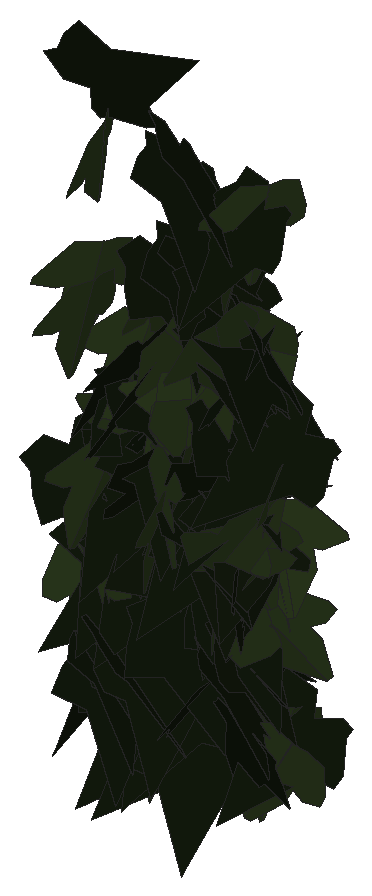
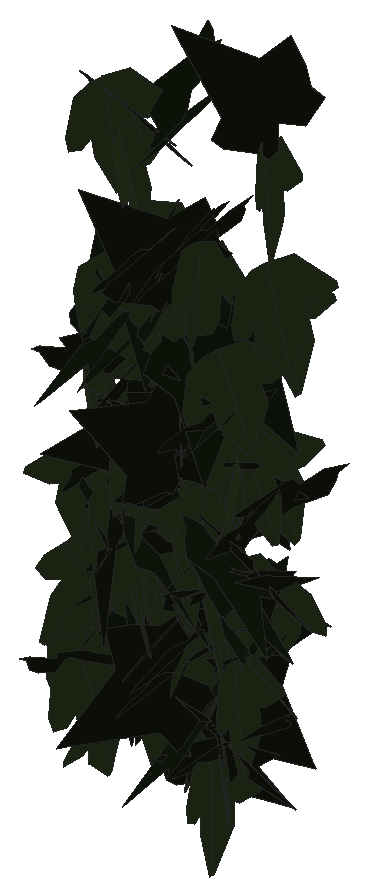
# SketchUp Ruby script. Lengths in inches.
U = 1.inch
M = Sketchup.active_model
def pt(a) = Geom::Point3d.new(a.map { |v| v * U })
def face(e, loops, mat)
  f = e.add_face(loops[0].map { |a| pt(a) })
  loops[1..].each { |l| e.add_face(l.map { |a| pt(a) }).erase! }
  f.material = f.back_material = mat if mat
  f
end
# faces: each face lists its corners as indices into pts; further lists are holes
def faces(e, pts, list, mat = nil) = list.each { |f| face(e, (f[0].is_a?(Array) ? f : [f]).map { |l| l.map { |i| pts[i] } }, mat) }
# xy, xz, yz: faces in a plane at the given z, y or x. An outline is a flat list of corners, or four numbers for a rectangle; further outlines are holes
def ring(l) = l.size == 4 ? [[l[0], l[1]], [l[2], l[1]], [l[2], l[3]], [l[0], l[3]]] : l.each_slice(2).to_a
def flat(e, list, mat, &to3) = list.each { |f| face(e, (f[0].is_a?(Array) ? f : [f]).map { |l| ring(l).map { |u, v| to3.(u, v) } }, mat) }
def xy(e, z, list, mat = nil) = flat(e, list, mat) { |x, y| [x, y, z] }
def xz(e, y, list, mat = nil) = flat(e, list, mat) { |x, z| [x, y, z] }
def yz(e, x, list, mat = nil) = flat(e, list, mat) { |y, z| [x, y, z] }
def lines(e, pts, list) = list.each { |a, b| e.add_line(pt(pts[a]), pt(pts[b])) }
# prism: a flat outline (further loops are holes) pulled along v
def prism(e, loops, v, mat = nil)
  f = face(e, loops, mat); d = Geom::Vector3d.new(v.map { |x| x * U })
  f.pushpull(f.normal.samedirection?(d) ? d.length : -d.length)
end
def box(e, o, s, mat = nil) = prism(e, [[o, [o[0] + s[0], o[1], o[2]], [o[0] + s[0], o[1] + s[1], o[2]], [o[0], o[1] + s[1], o[2]]]], [0, 0, s[2]], mat)
def at(x, y, z, deg = 0) = Geom::Transformation.translation(pt([x, y, z])) * Geom::Transformation.rotation(ORIGIN, Z_AXIS, deg.degrees)
def axes(o, x, y, z) = Geom::Transformation.new([*x, 0, *y, 0, *z, 0, *pt(o).to_a, 1])
def part(name) = M.definitions.add(name)
# library, detail: a bought-in or finely detailed component or shape, given as its bounding box
def library(name, o, s) = part(name).tap { |d| box(d.entities, o, s) }
def detail(e, o, s) = box(e.add_group.entities, o, s)
def put(e, d, t, mat = nil) = e.add_instance(d, t).tap { |i| i.material = mat if mat }
def group(e, t, mat = nil) = e.add_group.tap { |g| g.transformation = t; g.material = mat if mat }.entities
root = M.entities
M.materials.add("efeu1").color = [18, 25, 13]
M.materials.add("efeu2").color = [43, 57, 29]
c1 = part("ivyleaf_10")
p = [[0,0.5,-0.03],[-0.0625,2.02,-0.43],[-0.19,2.01,-0.46],[-0.54,1.05,-0.29],[-0.52,0.625,-0.18],[-0.83,0.76,-0.28],
  [-1.16,0.64,-0.33],[-1.15,0.33,-0.24],[-0.77,-0.39,0.02],[-0.3,-0.51,0.16],[0.04,-0.48,0.23],[-0.02,2.01,-0.4375],
  [-0.06,2.01,-0.43],[0.04,-0.49,0.23],[0.67,-0.49,0.14],[1.38,0.36,-0.2],[1.375,0.51,-0.24],[0.81,0.65,-0.19],
  [0.62,0.59,-0.15],[0.6,1.09,-0.28],[0.5,1.23,-0.31]]
faces(c1.entities,p,[[0,1,2,3,4,5,6,7,8,9,10],[11,12,0,13,14,15,16,17,18,19,20]],"efeu2")
c2 = part("ivyleaf_9")
p = [[1.54,2.16,1.25],[1.36,2.04,1.19],[-0.21,0.99,0.68],[-0.71,1.11,0.82],[-0.85,0.86,0.67],[-0.8,0.17,0.21],
  [-0.9,-0.01,0.1],[-0.67,-0.16,-0.02],[-0.08,-0.08,-0.05],[-0.03,-0.6,-0.4],[0.65,-0.88,-0.66],[0.83,-0.6,-0.49],
  [1.29,-0.42,-0.43],[1.8125,-0.07,-0.26],[1.21,0.44,0.15]]
faces(c2.entities,p,[[0,1,2,3,4,5,6,7,8,9,10,11,12,13,14]],"efeu1")
put(root,c1,axes([34.11,223.34,234.7],[0.03358,-0.4914,-0.086],[-0.00003,0.0862,-0.49251],[0.49887,0.03309,0.00576]))
put(root,c1,axes([34.14,222.76,239.2],[-0.18902,-0.45532,0.08338],[0.00238,-0.09102,-0.49164],[0.46289,-0.18546,0.03657]))
put(root,c2,axes([34.125,223.26,234.54],[-0.15536,0.18817,-0.43641],[0.22397,-0.37597,-0.24184],[-0.41916,-0.27063,0.03253]))
put(root,c2,axes([33.87,222.69,236.875],[0.17375,-0.38611,-0.26595],[0.02805,0.29168,-0.40514],[0.468,0.12586,0.12302]))
put(root,c1,axes([34.16,222.77,240.65],[0.12089,-0.4627,-0.14593],[-0.00592,0.14897,-0.47726],[0.48513,0.11712,0.03054]))
put(root,c2,axes([34.42,223.24,236.16],[-0.17172,0.43146,0.18535],[-0.15176,0.13578,-0.45666],[-0.44439,-0.21309,0.08432]))
put(root,c1,axes([34.19,222.53,238.87],[-0.0271,-0.49787,0.03732],[0.00573,-0.03768,-0.49855],[0.49923,-0.02659,0.00774]))
put(root,c1,axes([34.2,223.65,233.7],[0.00023,-0.48904,-0.10413],[0.02345,0.10403,-0.4885],[0.49945,-0.00466,0.02298]))
put(root,c2,axes([34.56,223.33,233.95],[-0.28419,0.24786,0.32834],[-0.27435,0.18318,-0.37574],[-0.30655,-0.39372,0.03188]))
put(root,c1,axes([34.41,222.93,237.19],[-0.43307,-0.01374,0.24952],[-0.24213,-0.1004,-0.42578],[0.0618,-0.48962,0.08031]))
put(root,c1,axes([34.23,223.51,234.2],[0.28638,-0.40282,-0.07567],[0.00576,0.09625,-0.49061],[0.40982,0.28013,0.05977]))
put(root,c1,axes([34.08,222.67,235.6],[0.47852,-0.03633,0.14036],[0.13956,-0.01571,-0.47987],[0.03928,0.49843,-0.0049]))
put(root,c2,axes([34.03,223.48,234.11],[0.07427,-0.47912,-0.12219],[0.08679,0.13427,-0.47375],[0.48678,0.04916,0.10311]))
put(root,c2,axes([34.5,223.35,236.12],[-0.39406,0.27061,-0.14658],[0.08038,-0.13938,-0.4734],[-0.29708,-0.39667,0.06634]))
put(root,c1,axes([34.36,222.62,236.94],[-0.08972,-0.4571,0.18168],[-0.00274,-0.18421,-0.46482],[0.49188,-0.0844,0.03055]))
put(root,c2,axes([34.11,223.26,236.59],[0.07666,-0.49409,0.00124],[0.00011,-0.00124,-0.5],[0.49409,0.07666,-0.00008]))
put(root,c2,axes([34.29,223.24,235.73],[-0.30239,-0.39405,0.05729],[0.056,-0.11331,-0.48376],[0.39424,-0.28615,0.11266]))
put(root,c1,axes([34.44,223.18,238.26],[-0.26244,-0.39372,0.16159],[-0.00493,-0.18701,-0.46368],[0.42556,-0.24497,0.09428]))
put(root,c2,axes([34.5625,223.14,235.54],[-0.38086,-0.25859,0.19513],[-0.15815,-0.11442,-0.46032],[0.28272,-0.41236,0.00536]))
put(root,c2,axes([34.56,223.5,233.75],[-0.4195,-0.25933,0.08226],[-0.05676,-0.06442,-0.49257],[0.26608,-0.42261,0.02461]))
put(root,c1,axes([34.51,223.36,235.55],[0.30708,-0.35032,-0.18159],[-0.09709,0.15595,-0.46503],[0.38246,0.32087,0.02776]))
put(root,c2,axes([34.75,223.04,236.17],[-0.48681,0.10802,0.03673],[-0.03736,0.00117,-0.4986],[-0.1078,-0.48819,0.00693]))
put(root,c1,axes([34.51,223.0625,236.9],[-0.38778,0.31246,0.04468],[-0.03268,0.03066,-0.49799],[-0.31394,-0.38914,-0.00335]))
put(root,c2,axes([34.11,222.76,241.23],[0.03647,-0.07809,0.49252],[0.46778,-0.16576,-0.06092],[0.17279,0.46522,0.06097]))
put(root,c2,axes([34.72,222.96,235.22],[-0.4416,0.2098,-0.10473],[0.08598,-0.06289,-0.48852],[-0.21816,-0.44947,0.01946]))
put(root,c2,axes([34.3125,222.74,234.62],[0.14282,-0.45162,0.16012],[0.06793,-0.14631,-0.47326],[0.47433,0.15694,0.01957]))
put(root,c2,axes([34.76,222.69,238.39],[-0.19998,0.38391,-0.25024],[0.05685,-0.25014,-0.42918],[-0.45473,-0.20011,0.05639]))
put(root,c2,axes([34.63,223.28,235.65],[-0.31388,-0.37861,0.0902],[0.01511,-0.12764,-0.4832],[0.38891,-0.3006,0.09157]))
put(root,c2,axes([34.69,222.86,236.79],[-0.4249,-0.2517,-0.07816],[0.07005,0.0351,-0.49382],[0.25408,-0.4306,0.00543]))
put(root,c2,axes([34.42,223.43,236.28],[0.04909,-0.47702,0.14157],[0.07836,-0.13307,-0.47556],[0.49138,0.06887,0.06169]))
put(root,c1,axes([34.67,223,234.7],[-0.20063,-0.44955,-0.08745],[0.07749,0.06078,-0.4902],[0.45138,-0.21025,0.04529]))
put(root,c2,axes([34.47,223.54,234.28],[0.37542,-0.29256,-0.1532],[-0.08783,0.13514,-0.47331],[0.31835,0.38229,0.05007]))
put(root,c2,axes([34.5625,222.63,234.59],[-0.04459,-0.49779,-0.01458],[0.00178,0.01448,-0.49979],[0.498,-0.04462,0.00048]))
put(root,c2,axes([34.48,223.23,234.26],[0.06732,-0.45206,0.20277],[0.083,-0.19145,-0.45438],[0.48845,0.09483,0.04926]))
put(root,c1,axes([34.6,223.14,236.6],[0.21448,0.43607,0.11765],[0.04232,0.11026,-0.48585],[-0.44967,0.21837,0.01039]))
put(root,c2,axes([34.6,223.01,237.6],[0.03646,-0.46071,-0.19083],[0.04023,0.19343,-0.45931],[0.49704,0.01813,0.05118]))
put(root,c1,axes([34.81,223.26,236.66],[0.4838,-0.10925,-0.06327],[-0.05445,0.0455,-0.49494],[0.1139,0.48579,0.03213]))
put(root,c2,axes([34.53,222.91,237.75],[0.28843,-0.40826,0.01141],[0.08787,0.04839,-0.48983],[0.39886,0.28457,0.09966]))
put(root,c2,axes([34.55,222.39,235.01],[0.39792,-0.29941,0.04482],[0.03562,-0.02722,-0.49799],[0.30065,0.39951,-0.00033]))
put(root,c1,axes([34.61,222.62,237.51],[-0.12944,-0.16385,-0.45431],[0.37363,0.26406,-0.20169],[0.30602,-0.3917,0.05408]))
put(root,c1,axes([35.01,222.91,235.2],[-0.47143,-0.05851,0.15599],[-0.13811,-0.12462,-0.46411],[0.09319,-0.48067,0.10134]))
put(root,c2,axes([34.96,221.96,237.88],[0.08046,0.31546,0.37949],[0.03899,0.37923,-0.32352],[-0.49194,0.08166,0.03643]))
put(root,c1,axes([34.98,222.88,239.2],[-0.0234,-0.47311,-0.16006],[0.00964,0.15978,-0.47369],[0.49936,-0.02526,0.00165]))
put(root,c2,axes([34.73,222.58,236.74],[0.24245,0.18452,0.39645],[0.29624,0.26412,-0.3041],[-0.32165,0.38235,0.01875]))
put(root,c2,axes([35.07,223.15,233.89],[-0.38153,-0.2921,0.13824],[-0.07227,-0.13135,-0.477],[0.31498,-0.38396,0.05801]))
put(root,c2,axes([35.09,223.14,237.37],[-0.06976,0.2846,-0.40513],[0.04835,-0.40327,-0.29162],[-0.49274,-0.07986,0.02874]))
put(root,c2,axes([35.17,222.66,237.82],[-0.03634,0.4743,0.154],[-0.07238,0.14776,-0.47215],[-0.4934,-0.05661,0.05792]))
put(root,c2,axes([34.77,223.41,235.01],[0.13319,-0.47341,-0.09026],[-0.00605,0.09199,-0.49143],[0.4819,0.132,0.01878]))
put(root,c2,axes([35.09,223.06,234.37],[-0.40654,-0.28505,-0.05895],[0.04738,0.03512,-0.49651],[0.2872,-0.40929,-0.00154]))
put(root,c1,axes([35.1,223.18,236.1],[0.46743,-0.01759,-0.17663],[-0.15297,0.21249,-0.42597],[0.09005,0.45226,0.19326]))
put(root,c1,axes([35.08,222.72,233.96],[0.13868,-0.35633,-0.32217],[-0.01819,0.33119,-0.37414],[0.48004,0.1155,0.07889]))
put(root,c1,axes([34.86,223.04,235.77],[0.28357,-0.32752,0.24963],[0.24765,-0.10654,-0.42109],[0.32903,0.36246,0.1018]))
put(root,c2,axes([34.8125,223.5,234.63],[0.42765,0.17333,0.19253],[0.1735,0.08432,-0.46129],[-0.19238,0.46135,0.01198]))
put(root,c2,axes([34.89,223.44,234.61],[0.09393,-0.4685,-0.14725],[-0.00409,0.14916,-0.47721],[0.49108,0.09085,0.02418]))
put(root,c1,axes([35.2,223.22,234.41],[-0.40893,-0.28756,-0.00917],[0.0055,0.00813,-0.4999],[0.28766,-0.40895,-0.00348]))
put(root,c1,axes([35.16,222.61,236.73],[0.19148,-0.4548,0.08061],[0.04294,-0.06935,-0.4933],[0.45988,0.19583,0.0125]))
put(root,c2,axes([35.01,223.38,237.2],[0.07138,-0.05001,0.49235],[0.35069,0.35609,-0.01467],[-0.34918,0.34741,0.08591]))
put(root,c1,axes([35.04,222.58,237.1],[-0.34113,0.24052,-0.27529],[0.16592,-0.23364,-0.40973],[-0.32573,-0.37089,0.07959]))
put(root,c1,axes([35.2,222.94,237.29],[0.22936,-0.41378,-0.16179],[-0.00212,0.18105,-0.46606],[0.44428,0.21448,0.0813]))
put(root,c2,axes([35.13,222.71,234.87],[-0.31475,-0.33373,-0.1989],[0.13584,0.14528,-0.45874],[0.36398,-0.34281,-0.00079]))
put(root,c2,axes([35.12,222.89,237.35],[-0.27304,-0.38906,-0.15519],[0.12237,0.10307,-0.47371],[0.40059,-0.29666,0.03894]))
put(root,c2,axes([35.49,223.23,236.07],[-0.34253,0.36424,0.0015],[-0.00669,-0.00424,-0.49994],[-0.36418,-0.34251,0.00778]))
put(root,c1,axes([35.33,223.25,235.84],[-0.33116,-0.36474,0.08542],[-0.0186,-0.09786,-0.48998],[0.37415,-0.3277,0.05125]))
put(root,c2,axes([35.12,222.92,236.1],[-0.14947,-0.43464,-0.19685],[0.06943,0.18428,-0.45959],[0.47206,-0.16472,0.00527]))
put(root,c2,axes([35.03,222.75,239.53],[0.18427,-0.43161,-0.1725],[-0.01394,0.18034,-0.46613],[0.4646,0.1766,0.05443]))
put(root,c1,axes([35.53,222.6875,238.05],[-0.3951,0.00452,0.3064],[-0.29003,-0.16686,-0.37154],[0.0989,-0.47131,0.13447]))
put(root,c2,axes([35.48,223.25,235.79],[-0.47885,-0.13396,0.0525],[-0.05066,-0.0138,-0.49724],[0.13467,-0.48152,-0.00035]))
put(root,c2,axes([35.06,223.27,235.0625],[0.19502,-0.45951,-0.02855],[0.00677,0.03386,-0.49881],[0.46035,0.19417,0.01943]))
put(root,c1,axes([35.39,223.29,236.17],[0.13846,-0.46313,-0.12785],[-0.00092,0.13279,-0.48204],[0.48045,0.13372,0.03592]))
put(root,c2,axes([35.17,223.07,239.39],[0.07597,-0.48494,0.09521],[-0.0029,-0.09677,-0.49054],[0.49419,0.07398,-0.01751]))
put(root,c2,axes([35.3,223.02,233.86],[-0.23079,-0.429,-0.11267],[0.08281,0.0831,-0.48604],[0.43575,-0.243,0.03269]))
put(root,c2,axes([35.21,223.16,234.57],[0.49727,-0.03058,-0.04225],[-0.04176,0.00925,-0.49817],[0.03125,0.49898,0.00664]))
put(root,c1,axes([35.38,222.49,238.8125],[-0.14094,-0.3639,-0.31259],[0.16426,0.2695,-0.3878],[0.45073,-0.21201,0.04358]))
put(root,c1,axes([35.54,222.81,235.83],[0.3514,-0.27279,-0.22825],[-0.10366,0.22839,-0.43254],[0.34025,0.35132,0.10396]))
put(root,c2,axes([35.54,223.03,236.4375],[-0.43177,-0.25164,-0.01603],[0.06393,-0.0785,-0.48964],[0.24391,-0.42487,0.09996]))
put(root,c1,axes([35.44,223.37,235.26],[0.3071,-0.39402,0.02088],[0.0456,0.00916,-0.49783],[0.39193,0.30767,0.04156]))
put(root,c1,axes([35.37,222.5,238.11],[-0.03035,-0.1272,-0.48259],[0.27004,0.40241,-0.12305],[0.41971,-0.26811,0.04427]))
put(root,c2,axes([35.71,223.09,237.34],[-0.47637,-0.15158,0.00989],[-0.00928,-0.00346,-0.4999],[0.15162,-0.47646,0.00049]))
put(root,c2,axes([35.33,222.92,239.02],[-0.10944,-0.07824,0.48156],[0.47076,0.11265,0.12529],[-0.1281,0.48082,0.04901]))
put(root,c2,axes([35.45,223.3,236],[-0.09988,-0.48477,0.07083],[0.00562,-0.07342,-0.49455],[0.48989,-0.09799,0.02012]))
put(root,c2,axes([35.17,223.23,234.93],[0.27037,-0.243,0.34329],[0.26826,-0.21469,-0.36324],[0.32395,0.3806,0.01428]))
put(root,c2,axes([35.4,222.58,235.47],[0.03156,-0.45448,-0.20603],[0.03565,0.20797,-0.4533],[0.49773,0.01392,0.04554]))
put(root,c2,axes([35.36,223.24,235.09],[0.26801,-0.3956,-0.14722],[-0.01015,0.16829,-0.47072],[0.42198,0.25531,0.08218]))
put(root,c2,axes([35.38,222.68,240.68],[0.05009,-0.46932,0.16501],[0.08782,-0.1549,-0.46722],[0.48967,0.07579,0.06691]))
put(root,c2,axes([35.8125,222.49,234.89],[-0.19665,0.45294,-0.07859],[0.02413,-0.07519,-0.49372],[-0.45907,-0.19797,0.00772]))
put(root,c1,axes([35.68,223.2,236.73],[0.05466,-0.49654,-0.02149],[-0.01417,0.02005,-0.4994],[0.4968,0.0552,-0.01188]))
put(root,c2,axes([35.3,222.89,236.48],[0.21085,-0.42989,0.144],[0.1583,-0.07901,-0.46765],[0.42483,0.2428,0.10278]))
put(root,c1,axes([36.05,223.23,238.57],[-0.08394,-0.00248,-0.4929],[-0.477,-0.12558,0.08186],[-0.1242,0.48397,0.01871]))
put(root,c2,axes([35.89,223.36,236.14],[0.1905,0.03593,-0.46089],[-0.45956,0.06874,-0.1846],[0.0501,0.49395,0.05921]))
put(root,c1,axes([35.76,223.25,236.39],[-0.12369,-0.4558,0.16417],[0.01058,-0.17193,-0.46939],[0.48434,-0.11265,0.05218]))
put(root,c2,axes([35.42,222.55,241.02],[0.25946,-0.38335,0.18901],[0.1003,-0.16032,-0.46286],[0.41547,0.2781,-0.00629]))
put(root,c2,axes([35.63,223.01,236.54],[-0.12405,-0.46902,-0.12095],[0.04812,0.11231,-0.48484],[0.48197,-0.13193,0.01727]))
put(root,c1,axes([35.875,222.76,236.67],[-0.4902,0.04785,0.0861],[-0.09629,-0.14065,-0.47005],[-0.02076,-0.47742,0.1471]))
put(root,c1,axes([35.71,223.5625,233.9375],[-0.01299,0.48038,-0.13807],[-0.00656,-0.13827,-0.48046],[-0.49979,-0.01067,0.00989]))
put(root,c2,axes([35.54,223.06,239.28],[0.15007,-0.4533,-0.14833],[0.01567,0.1601,-0.47342],[0.47669,0.13744,0.06226]))
put(root,c2,axes([35.46,222.67,236.94],[0.29975,0.11694,0.38272],[0.34263,0.17207,-0.32093],[-0.20677,0.45466,0.02302]))
put(root,c1,axes([35.72,223.05,235.97],[0.36094,-0.32374,0.12214],[0.08174,-0.09173,-0.48467],[0.33622,0.36984,-0.01329]))
put(root,c2,axes([36.0625,222.56,238.41],[-0.07122,0.41135,0.27517],[-0.09393,0.26172,-0.41555],[-0.48591,-0.11088,0.04]))
put(root,c2,axes([35.98,222.85,236.18],[0.11385,-0.05936,-0.48323],[-0.42227,0.23497,-0.12835],[0.24233,0.43734,0.00337]))
put(root,c2,axes([35.68,222.69,238.64],[0.42435,-0.16301,-0.20821],[-0.15674,0.16203,-0.4463],[0.21297,0.44404,0.08641]))
put(root,c2,axes([35.91,223.05,237.21],[-0.45598,-0.11059,-0.17277],[0.19559,-0.10745,-0.44744],[0.06184,-0.47563,0.14125]))
put(root,c2,axes([35.64,223.1875,235.49],[0.09036,-0.48578,-0.07651],[0.08791,0.09249,-0.48344],[0.48385,0.07392,0.10212]))
put(root,c1,axes([35.96,223.16,235.82],[-0.03905,-0.45391,-0.20601],[0.02519,0.20458,-0.45554],[0.49784,-0.04595,0.00689]))
put(root,c1,axes([36.01,222.39,239.11],[-0.12783,-0.45508,-0.16298],[0.03207,0.16022,-0.47255],[0.48232,-0.13126,-0.01178]))
put(root,c2,axes([35.76,222.89,237.81],[0.21009,-0.43728,-0.12104],[-0.0273,0.12096,-0.48438],[0.4529,0.21014,0.02695]))
put(root,c1,axes([36.03,222.8,240.16],[0.15394,-0.47571,-0.00042],[0.00298,0.0014,-0.49999],[0.4757,0.15393,0.00327]))
put(root,c2,axes([36.21,223.04,236.11],[-0.38319,0.30335,-0.10557],[0.08986,-0.05654,-0.4886],[-0.30837,-0.39342,-0.01119]))
put(root,c2,axes([35.79,223.08,235.18],[0.27184,-0.40706,-0.10202],[-0.04567,0.09213,-0.48931],[0.41715,0.27535,0.01291]))
put(root,c2,axes([35.98,223.16,236.67],[-0.18664,-0.46177,0.04398],[-0.00048,-0.04722,-0.49777],[0.46386,-0.18585,0.01718]))
put(root,c2,axes([35.83,223.2,238.47],[0.39276,-0.2591,-0.16914],[-0.09366,0.16094,-0.46403],[0.2949,0.39619,0.07789]))
put(root,c1,axes([36.14,223.36,234.12],[-0.17326,-0.45238,0.12382],[-0.01504,-0.12657,-0.48348],[0.46878,-0.17126,0.03025]))
put(root,c1,axes([36.0625,222.77,235.48],[0.05471,-0.20049,0.45476],[-0.07686,0.44859,0.20702],[-0.49102,-0.09256,0.01827]))
put(root,c1,axes([36.09,222.67,236.62],[-0.36468,-0.3089,-0.14695],[0.1142,0.09253,-0.47791],[0.32244,-0.38213,0.00307]))
put(root,c1,axes([36.05,223.24,235.41],[-0.35274,-0.23329,-0.26674],[0.21681,0.15561,-0.42282],[0.2803,-0.41395,-0.00862]))
put(root,c2,axes([36.3,222.43,234.49],[0.29551,0.10361,-0.38979],[-0.38708,-0.06291,-0.31018],[-0.11332,0.48509,0.04303]))
put(root,c1,axes([36.05,222.56,236.4],[-0.26492,-0.37221,0.20317],[0.17316,0.12372,0.45245],[-0.38709,0.31008,0.06335]))
put(root,c2,axes([36.03,223.24,238.54],[-0.06121,-0.20039,0.45398],[0.16839,-0.43867,-0.17092],[0.46679,0.13197,0.12119]))
put(root,c1,axes([36.17,223.19,236.5625],[0.36389,0.32989,0.09355],[0.03551,0.09943,-0.48873],[-0.34106,0.36233,0.04893]))
put(root,c1,axes([36.35,222.75,240.65],[-0.18862,-0.45949,0.05734],[0.01202,-0.06676,-0.49538],[0.4629,-0.1855,0.03623]))
put(root,c2,axes([36.05,222.76,238.76],[0.04886,-0.41764,0.27053],[0.13652,-0.25015,-0.41084],[0.47851,0.11401,0.08959]))
put(root,c2,axes([35.99,222.64,234.89],[0.1633,-0.37153,0.29205],[0.16539,-0.24453,-0.40355],[0.4427,0.2284,0.04303]))
put(root,c1,axes([36.32,223.03,237.3],[0.23641,-0.44042,-0.01177],[0.01527,0.02154,-0.4993],[0.44031,0.23572,0.02364]))
put(root,c1,axes([36.55,222.85,234.13],[-0.41423,-0.10539,0.25943],[-0.23713,-0.11437,-0.42508],[0.14894,-0.4752,0.04477]))
put(root,c2,axes([36.42,222.58,240.61],[-0.47223,-0.05356,-0.15532],[0.16304,-0.09438,-0.46315],[0.0203,-0.48808,0.1066]))
put(root,c2,axes([36.41,223.42,234.24],[-0.41579,-0.27111,0.06018],[0.02123,-0.13906,-0.4798],[0.2769,-0.39644,0.12715]))
put(root,c2,axes([36.53,223.11,237.78],[-0.44176,-0.20717,0.10923],[-0.06521,-0.11517,-0.48216],[0.22494,-0.44025,0.07474]))
